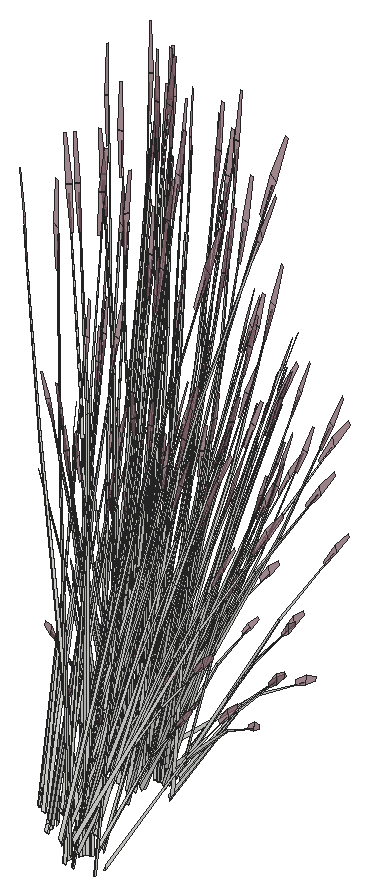
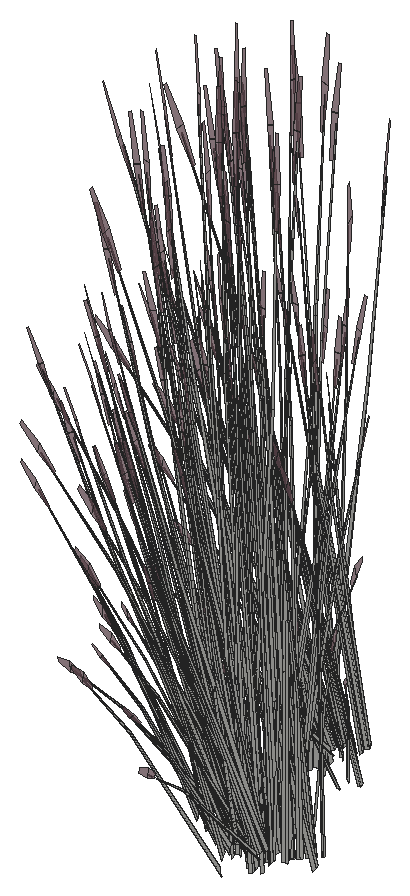
# SketchUp Ruby script. Lengths in inches.
U = 1.inch
M = Sketchup.active_model
def pt(a) = Geom::Point3d.new(a.map { |v| v * U })
def face(e, loops, mat)
  f = e.add_face(loops[0].map { |a| pt(a) })
  loops[1..].each { |l| e.add_face(l.map { |a| pt(a) }).erase! }
  f.material = f.back_material = mat if mat
  f
end
# faces: each face lists its corners as indices into pts; further lists are holes
def faces(e, pts, list, mat = nil) = list.each { |f| face(e, (f[0].is_a?(Array) ? f : [f]).map { |l| l.map { |i| pts[i] } }, mat) }
# xy, xz, yz: faces in a plane at the given z, y or x. An outline is a flat list of corners, or four numbers for a rectangle; further outlines are holes
def ring(l) = l.size == 4 ? [[l[0], l[1]], [l[2], l[1]], [l[2], l[3]], [l[0], l[3]]] : l.each_slice(2).to_a
def flat(e, list, mat, &to3) = list.each { |f| face(e, (f[0].is_a?(Array) ? f : [f]).map { |l| ring(l).map { |u, v| to3.(u, v) } }, mat) }
def xy(e, z, list, mat = nil) = flat(e, list, mat) { |x, y| [x, y, z] }
def xz(e, y, list, mat = nil) = flat(e, list, mat) { |x, z| [x, y, z] }
def yz(e, x, list, mat = nil) = flat(e, list, mat) { |y, z| [x, y, z] }
def lines(e, pts, list) = list.each { |a, b| e.add_line(pt(pts[a]), pt(pts[b])) }
# prism: a flat outline (further loops are holes) pulled along v
def prism(e, loops, v, mat = nil)
  f = face(e, loops, mat); d = Geom::Vector3d.new(v.map { |x| x * U })
  f.pushpull(f.normal.samedirection?(d) ? d.length : -d.length)
end
def box(e, o, s, mat = nil) = prism(e, [[o, [o[0] + s[0], o[1], o[2]], [o[0] + s[0], o[1] + s[1], o[2]], [o[0], o[1] + s[1], o[2]]]], [0, 0, s[2]], mat)
def at(x, y, z, deg = 0) = Geom::Transformation.translation(pt([x, y, z])) * Geom::Transformation.rotation(ORIGIN, Z_AXIS, deg.degrees)
def axes(o, x, y, z) = Geom::Transformation.new([*x, 0, *y, 0, *z, 0, *pt(o).to_a, 1])
def part(name) = M.definitions.add(name)
# library, detail: a bought-in or finely detailed component or shape, given as its bounding box
def library(name, o, s) = part(name).tap { |d| box(d.entities, o, s) }
def detail(e, o, s) = box(e.add_group.entities, o, s)
def put(e, d, t, mat = nil) = e.add_instance(d, t).tap { |i| i.material = mat if mat }
def group(e, t, mat = nil) = e.add_group.tap { |g| g.transformation = t; g.material = mat if mat }.entities
root = M.entities
M.materials.add("LightPink_Translucent").color = [144, 107, 117]
M.materials["LightPink_Translucent"].alpha = 0.75
c1 = part("blade")
p = [[2.15,0.21,22],[0,0.17,0],[0.09,0.45,0],[2.18,0.31,22],[2.29,0.31,22],[0.38,0.45,0],
  [2.48,0.24,33],[2.49,0.24,33],[2.48,0.22,33]]
faces(c1.entities,p,[[0,1,2,3],[4,5,2,3],[6,3,4,7],[8,0,3,6]])
c2 = part("seeds")
p = [[0.3,-0.1,1.38],[-0.01,-0.03,1.59],[-0.01,-0.03,0.03],[0.14,-0.07,-0.07],[0.29,-0.03,3],[0.15,0.01,3.11]]
faces(c2.entities,p,[[0,1,2,3],[1,0,4,5]],"LightPink_Translucent")
c3 = part("blade with seeds")
put(c3.entities,c1,at(0,0,0))
put(c3.entities,c2,axes([2.4,0.25,30.99],[1.5799,-0.05474,1.17369],[-0.12525,1.92788,0.29478],[-0.07173,-0.02425,1.56792]))
put(root,c3,axes([299.23,498.21,2.21],[-0.43405,0.58792,-0.44739],[-0.90188,-0.28295,0.21531],[0,0.13553,1.43643]))
put(root,c3,axes([301.09,499.59,4.73],[-0.65964,0.42992,0.48003],[-0.5689,-0.45657,0.3958],[0.30948,0.0793,0.9933]))
put(root,c3,axes([298.99,500.09,5.05],[-0.13817,-0.52554,0.35414],[0.78985,-0.13877,-0.4572],[0.21215,0.1506,0.87481]))
put(root,c3,axes([299.26,499.89,2.33],[1.11998,0.21207,0.30756],[-0.2802,0.75803,-0.36492],[-0.18537,0.09487,1.64885]))
put(root,c3,axes([299.18,500.41,2.02],[-0.83726,0.32623,-0.49651],[-0.50045,-0.58498,0],[-0.19069,0.0743,1.57504]))
put(root,c3,axes([301.96,498.47,2.02],[0,0.65246,-0.49651],[-1.00089,0,0],[0,0.1486,1.57504]))
put(root,c3,axes([299.46,498.55,3.875],[-0.3323,-0.11241,1.71376],[0.68769,-0.4716,0.13857],[0.42861,0.21275,0.73262]))
put(root,c3,axes([299.52,497.07,4.47],[-0.77304,-0.33901,1.38283],[0.81626,-0.52782,0.59665],[0.24941,0.31809,1.33663]))
put(root,c3,axes([300.6875,499.83,2.77],[-0.5037,-0.18761,1.1486],[0.6504,-0.19062,0.84392],[0.17543,0.16147,0.25299]))
put(root,c3,axes([298.92,500.36,5.03],[0.53309,-0.55848,-0.1216],[0.77201,0.32175,-0.67495],[0.26836,0.15779,1.02557]))
put(root,c3,axes([295.4,499.61,5.05],[0.60531,-0.34352,0.35414],[0.573,0.39225,-0.4572],[-0.08718,0.19929,0.87481]))
put(root,c3,axes([299.9375,500.3,2.375],[0.55932,0.6538,0],[-0.93577,0.36461,-0.51607],[-0.21313,0.08304,1.63711]))
put(root,c3,axes([298.22,500.83,4.71],[0.00265,-0.07899,1.77383],[0.76665,-0.34851,-0.16761],[0.2663,0.12439,0.31391]))
put(root,c3,axes([300.83,500.52,1.49],[0.06518,-0.0942,1.76342],[0.82057,-0.27742,-0.26939],[0.24877,0.14358,0.30037]))
put(root,c3,axes([299.46,497.72,2.84],[-0.02444,-0.61432,1.41272],[1.10603,0.15924,0.59816],[-0.26159,0.33615,1.3335]))
put(root,c3,axes([299.74,498.38,2.09],[0.32803,0.59738,-0.69212],[-0.94492,0.21515,-0.18165],[0.03626,0.20229,1.52773]))
put(root,c3,axes([299.55,500.09,4.68],[0.88277,-0.1551,-0.51099],[0.15442,0.58737,-0.3958],[0.23711,0.16832,0.97773]))
put(root,c3,axes([297.1,500.17,5.05],[0.2697,-0.50175,0.35414],[0.78684,0.14635,-0.4572],[0.07215,0.20201,0.87481]))
put(root,c3,axes([300.77,500.68,2.67],[-0.57368,-0.02046,1.0506],[0.37886,-0.43461,0.58006],[0.22663,0.15441,0.8241]))
put(root,c3,axes([299.11,500.57,4.73],[-0.4066,0.41448,0.0643],[-0.57901,-0.24131,0.50621],[0.18719,0.13288,0.77189]))
put(root,c3,axes([298.16,501.96,5.65],[0.61821,-0.37431,-0.06488],[0.56645,0.40995,-0.29416],[0.03988,0.11616,0.97024]))
put(root,c3,axes([299.28,500.45,4.73],[-0.88979,0.14973,0.48003],[-0.15442,-0.58737,0.3958],[0.20926,0.17311,0.9933]))
put(root,c3,axes([298.89,499.63,2.59],[0.01579,-0.21629,1.43002],[0.75442,-0.24159,-0.30754],[0.23289,0.25887,0.61141]))
put(root,c3,axes([296.85,500.63,4.73],[-0.6592,0.22175,0.0643],[-0.32265,-0.40436,0.50621],[0.06366,0.17825,0.77189]))
put(root,c3,axes([295.02,499.7,5.4],[0.98321,0.03233,-0.13498],[-0.02687,0.61208,-0.74919],[-0.0683,0.23574,1.13838]))
put(root,c3,axes([296.84,500.39,5.03],[0.87543,-0.30377,-0.1216],[0.4302,0.53915,-0.67495],[0.1155,0.2272,1.02557]))
put(root,c3,axes([294.42,509.26,2.59],[-0.25429,0.13207,1.43002],[-0.76157,-0.23115,-0.30754],[0.14117,-0.28747,0.61141]))
put(root,c3,axes([297.09,500.59,5.0625],[-0.88151,-0.17057,0.53283],[0.30143,-0.56078,0.43934],[0.05297,0.22053,1.10256]))
put(root,c3,axes([295.47,501.43,2.77],[-0.02315,-0.38796,1.1486],[0.57853,0.27671,0.84392],[-0.11378,0.18492,0.25299]))
put(root,c3,axes([296.99,500.5,1.49],[0.14478,-0.0355,1.76342],[0.8709,0.19542,-0.26939],[0.02547,0.22025,0.30037]))
put(root,c3,axes([295.6875,499.93,5],[0.64041,0.4384,-0.5672],[-0.67652,0.38394,-0.43934],[-0.09744,0.22274,1.08528]))
put(root,c3,axes([295.04,510.24,4.98],[0.02328,-0.60353,-0.71045],[0.98022,0.04053,0.08574],[0.10344,-0.25568,1.00501]))
put(root,c3,axes([294.99,500.59,2.82],[0.8127,-0.11554,0.06507],[0.18684,0.46549,-0.86304],[-0.05152,0.23564,0.7736]))
put(root,c3,axes([297.59,500.36,4.68],[0.87941,0.16356,-0.51099],[-0.30143,0.56078,-0.3958],[0.08064,0.22578,0.97773]))
put(root,c3,axes([298.09,499.2,3.875],[-0.2045,-0.20949,1.71376],[0.94495,-0.17636,0.13857],[0.21357,0.32887,0.73262]))
put(root,c3,axes([296.4,509.3,4.72],[-0.00864,-0.12985,1.74944],[-0.72937,-0.3753,-0.27667],[0.11277,-0.2275,0.14031]))
put(root,c3,axes([293.93,509.93,3.875],[-0.16657,0.22426,1.71376],[-0.69879,-0.4641,0.13857],[0.31524,-0.28926,0.73262]))
put(root,c3,axes([296.21,508.83,4.71],[-0.09085,0.04984,1.77383],[-0.89014,-0.16814,-0.16761],[-0.03222,-0.21748,0.31391]))
put(root,c3,axes([297.1875,500.7,4.53],[-0.2697,0.50175,-0.35414],[-0.78684,-0.14635,0.4572],[0.07215,0.20201,0.87481]))
put(root,c3,axes([293.48,508.21,2.77],[0.11476,0.38047,1.1486],[-0.63664,-0.21072,0.84392],[0.06851,-0.19481,0.25299]))
put(root,c3,axes([295.49,499.73,5.34],[-0.02328,0.60353,-0.7886],[-0.98022,-0.04053,0.09517],[-0.10344,0.25568,1.11556]))
put(root,c3,axes([294.84,510.04,4.68],[-0.64041,-0.4384,-0.51099],[0.67652,-0.38394,-0.3958],[0.09744,-0.22274,0.97773]))
put(root,c3,axes([296.42,499.3,3.875],[-0.0219,-0.25042,1.71376],[0.94901,0.16613,0.13857],[-0.0587,0.35688,0.73262]))
put(root,c3,axes([297.27,500.25,4.98],[0.42698,0.53052,-0.71045],[-0.87893,0.29566,0.08574],[0.09984,0.25633,1.00501]))
put(root,c3,axes([293.4375,509.39,4.73],[0.88151,0.17057,0.48003],[-0.30143,0.56078,0.3958],[-0.05297,-0.22053,0.9933]))
put(root,c3,axes([295.51,510.27,5.03],[-0.98321,-0.03233,-0.1216],[0.02687,-0.61208,-0.67495],[0.0683,-0.23574,1.02557]))
put(root,c3,axes([295.44,509.875,4.53],[0.60531,-0.34352,-0.35414],[0.573,0.39225,0.4572],[0.08718,-0.19929,0.87481]))
put(root,c3,axes([293.67,509.34,4.73],[0.6592,-0.22175,0.0643],[0.32265,0.40436,0.50621],[-0.06366,-0.17825,0.77189]))
put(root,c3,axes([296.63,501.59,4.72],[0.1134,0.10507,1.74944],[0.91515,0.04128,-0.27667],[0.09203,0.23172,0.14031]))
put(root,c3,axes([295.16,500.58,3.36],[0.01966,-0.33682,1.54345],[0.88405,0.17791,0.21329],[-0.0766,0.35897,0.72882]))
put(root,c3,axes([296.2,509.67,1.49],[-0.1339,-0.0514,1.76342],[-0.34394,-0.57425,-0.26939],[0.23202,-0.15583,0.30037]))
put(root,c3,axes([295.4375,510.01,4.73],[0.63704,0.44518,0.48003],[-0.67652,0.38394,0.3958],[0.11751,-0.20886,0.9933]))
put(root,c3,axes([295.67,510.05,4.73],[0.73517,0.0304,0.0643],[-0.02016,0.45906,0.50621],[0.07693,-0.17585,0.77189]))
put(root,c3,axes([295.125,510.36,5.05],[-0.60531,0.34352,0.35414],[-0.573,-0.39225,-0.4572],[0.08718,-0.19929,0.87481]))
put(root,c3,axes([296.19,511.29,4.98],[0.4673,-0.51481,-0.71045],[0.81887,0.36587,0.08574],[0.27902,-0.18652,1.00501]))
put(root,c3,axes([291.14,509.79,2.375],[-0.55932,-0.6538,0],[0.93577,-0.36461,-0.51607],[0.21313,-0.08304,1.63711]))
put(root,c3,axes([296.17,511.05,4.68],[-0.22982,-0.59576,-0.51099],[0.87033,-0.10422,-0.3958],[0.24941,-0.16002,0.97773]))
put(root,c3,axes([296.58,511.47,5.03],[-0.82753,-0.35977,-0.1216],[0.47675,-0.52101,-0.67495],[0.2338,-0.18111,1.02557]))
put(root,c3,axes([291.9,509.6875,2.02],[0.83726,-0.32623,-0.49651],[0.50045,0.58498,0],[0.19069,-0.0743,1.57504]))
put(root,c3,axes([296.87,510.82,2.59],[-0.31959,-0.01933,1.43002],[-0.32741,-0.51843,-0.30754],[0.39262,-0.14666,0.61141]))
put(root,c3,axes([298.62,511.32,4.71],[-0.11685,-0.00496,1.77383],[-0.48522,-0.53096,-0.16761],[0.19486,-0.17458,0.31391]))
put(root,c3,axes([292.89,511.03,2.06],[0.60257,-0.49041,-0.62353],[0.74854,0.44469,-0.16365],[0.24146,-0.12234,1.37633]))
put(root,c3,axes([297.24,509.86,2.77],[-0.29798,0.33213,1.1486],[-0.25612,-0.44624,0.84392],[0.24611,-0.11182,0.25299]))
put(root,c3,axes([296.8125,511.11,4.53],[0.77872,-0.09325,-0.35414],[0.20563,0.53305,0.4572],[0.22316,-0.14318,0.87481]))
put(root,c3,axes([292.24,511.59,2.67],[-0.10425,-0.7445,-0.29095],[1.08575,-0.04502,-0.50002],[0.19119,-0.09917,1.59708]))
put(root,c3,axes([296.18,511.43,5.05],[-0.77872,0.09325,0.35414],[-0.20563,-0.53305,-0.4572],[0.22316,-0.14318,0.87481]))
put(root,c3,axes([292.1,509.95,2.03],[0.83462,0.16144,-0.30978],[-0.21015,0.56852,0.30978],[0.16826,-0.06556,1.38974]))
put(root,c3,axes([296.88,511.34,4.73],[0.61415,0.2744,0.0643],[-0.35756,0.39076,0.50621],[0.1969,-0.12633,0.77189]))
put(root,c3,axes([296.71,511.23,4.73],[0.22187,0.60049,0.48003],[-0.87033,0.10422,0.3958],[0.25651,-0.14123,0.9933]))
put(root,c3,axes([299.06,511.95,4.72],[0.12414,-0.09938,1.74944],[-0.15889,-0.60963,-0.27667],[0.31148,-0.11559,0.14031]))
put(root,c3,axes([292.38,512.18,2.43],[1.00799,0.31623,0.24065],[-0.48511,0.65709,0.50002],[0,-0.15147,1.60543]))
put(root,c3,axes([292.06,511.74,2.72],[-0.97146,0.04028,0.44739],[-0.08785,-0.66859,-0.21531],[0.17391,-0.06776,1.43643]))
put(root,c3,axes([296.61,512.88,5.03],[-0.45012,-0.59081,-0.1216],[0.79888,-0.29033,-0.67495],[0.33665,-0.07795,1.02557]))
put(root,c3,axes([296.57,512.37,4.68],[0.24236,-0.59349,-0.51099],[0.83094,0.20343,-0.3958],[0.33455,-0.05442,0.97773]))
put(root,c3,axes([295.26,509.95,2.375],[0.55932,-0.6538,0],[0.93577,0.36461,-0.51607],[0.21313,0.08304,1.63711]))
put(root,c3,axes([297.46,512.54,1.98],[-0.57619,0.0783,1.41583],[-0.09171,-0.62326,0.08104],[0.40356,-0.09434,0.80566]))
put(root,c3,axes([298.51,511.99,2.26],[-0.55463,-0.41721,-0.06488],[0.60744,-0.38228,-0.29416],[0.17212,-0.02691,0.97024]))
put(root,c3,axes([293.42,512.04,2.21],[0,-0.75495,0],[1.11865,0,0],[0,0,1.79456]))
put(root,c3,axes([294.78,510.3,2.48],[-0.83726,-0.32623,0.49651],[0.50045,-0.58498,0],[0.19069,0.0743,1.57504]))
put(root,c3,axes([296.41,512.59,4.98],[0.78611,-0.28816,-0.71045],[0.4381,0.59317,0.08574],[0.37982,-0.06738,1.00501]))
put(root,c3,axes([292.89,511.56,2.36],[-0.74176,0.59212,0.45755],[-0.88124,-0.52269,0.17955],[0.17882,-0.05909,1.58856]))
put(root,c3,axes([291.6,510.59,2.47],[-0.25843,0.64844,0.17642],[-0.9457,-0.1835,0.35086],[0.16336,-0.00316,1.60407]))
put(root,c3,axes([296.3,512.7,5.05],[-0.74348,-0.18202,0.35414],[0.21685,-0.53102,-0.4572],[0.29933,-0.04869,0.87481]))
put(root,c3,axes([291.21,511.11,1.59],[-0.88056,0.26122,1.28929],[-0.28027,-0.74951,0.50096],[0.54072,0.01247,1.46642]))
put(root,c3,axes([293.58,511.3125,2.62],[0.17258,-0.58229,0.1448],[0.84319,0.10108,-0.41347],[0.15345,0.05979,1.26744]))
put(root,c3,axes([298.09,512.13,1.49],[-0.04675,-0.09906,1.76342],[0.32428,-0.57943,-0.26939],[0.32711,-0.00833,0.30037]))
put(root,c3,axes([293.22,511.46,2.72],[-0.53742,-0.54764,0.44739],[0.81403,-0.38564,-0.21531],[0.17391,0.06776,1.43643]))
put(root,c3,axes([293.49,511.5,2.67],[0.90324,-0.43318,-0.29095],[0.60064,0.61207,-0.50002],[0.22285,0.06216,1.59708]))
put(root,c3,axes([297.08,512.64,4.53],[0.74348,0.18202,-0.35414],[-0.21685,0.53102,0.4572],[0.29933,-0.04869,0.87481]))
put(root,c3,axes([295.77,510.35,2.02],[0.83726,0.32623,-0.49651],[-0.50045,0.58498,0],[0.19069,0.0743,1.57504]))
put(root,c3,axes([294.18,512.21,2.21],[1.00089,0,0],[0,0.67548,0],[0,0,1.78407]))
put(root,c3,axes([294.46,510.625,2.47],[-0.96132,0.17317,0.17642],[-0.23737,-0.64447,0.35086],[0.08574,0.0939,1.60407]))
put(root,c3,axes([295.06,511.98,3.875],[-0.37107,0.01478,1.71376],[0.24616,-0.64047,0.13857],[0.5288,0.03961,0.73262]))
put(root,c3,axes([295.54,510.59,2.03],[0.21015,0.56852,-0.30978],[-0.83462,0.16144,0.30978],[0.16826,0.06556,1.38974]))
put(root,c3,axes([296.97,512.87,4.73],[0.32857,0.44488,0.0643],[-0.59916,0.21775,0.50621],[0.26412,-0.04296,0.77189]))
put(root,c3,axes([293.86,511.87,2.38],[-1.13071,-0.13747,0.49198],[0.23011,-0.77639,0.19306],[0.16524,0.07497,1.70813]))
put(root,c3,axes([296.91,512.71,4.73],[-0.25275,0.59491,0.48003],[-0.83094,-0.20343,0.3958],[0.32677,-0.03575,0.9933]))
put(root,c3,axes([294.05,513.7,2.18],[0.93921,-0.22138,-0.19198],[0.33003,0.6377,0.00008],[0.10367,-0.02447,1.73897]))
put(root,c3,axes([294.16,512.5,2.21],[0.62448,0.42144,0],[-0.62448,0.42144,0],[0,0,1.69266]))
put(root,c3,axes([295.85,512.32,2.47],[-0.70288,-0.47526,0.17642],[0.70832,-0.46097,0.35086],[-0.07763,0.09706,1.60407]))
put(root,c3,axes([294.55,511.6,2.06],[0.9306,0.10697,-0.62353],[-0.19638,0.65984,-0.16365],[0.27771,0.07995,1.37633]))
put(root,c3,axes([298.66,512.75,2.77],[-0.55274,0.10771,1.1486],[0.26018,-0.44517,0.84392],[0.29323,0.03046,0.25299]))
put(root,c3,axes([294.15,512.01,2.72],[0.43405,-0.58792,0.44739],[0.90188,0.28295,-0.21531],[0,0.13553,1.43643]))
put(root,c3,axes([298.4,514.63,4.71],[-0.08089,-0.05712,1.77383],[0.17695,-0.61228,-0.16761],[0.31864,-0.03912,0.31391]))
put(root,c3,axes([293.98,512.34,2.29],[0,0.75458,-0.05637],[-1.11865,0,0],[0,0.02371,1.79368]))
put(root,c3,axes([294.06,511.81,2.21],[0.53742,0.54764,-0.44739],[-0.81403,0.38564,0.21531],[0.17391,0.06776,1.43643]))
put(root,c3,axes([297.7,514.12,3.93],[-0.17122,-0.54847,-0.03492],[0.80929,-0.12609,-0.15832],[0.169,0.03477,0.52218]))
put(root,c3,axes([295.6,514.11,5.03],[0.0479,-0.66354,-0.1216],[0.90696,0.01814,-0.67495],[0.3493,0.04609,1.02557]))
put(root,c3,axes([296.43,512.33,2.48],[0,-0.65246,0.49651],[1.00089,0,0],[0,0.1486,1.57504]))
put(root,c3,axes([294.53,512.14,2.62],[0.83351,-0.19028,0.1448],[0.29189,0.54335,-0.41347],[0,0.11958,1.26744]))
put(root,c3,axes([295.46,513.85,5.05],[-0.50902,-0.40851,0.35414],[0.58122,-0.38671,-0.4572],[0.29531,0.05884,0.87481]))
put(root,c3,axes([297.625,513.46,2.59],[-0.21545,-0.16047,1.43002],[0.28033,-0.53085,-0.30754],[0.43591,0.07191,0.61141]))
put(root,c3,axes([293.77,514.05,2.2],[0.90188,0.29293,0],[-0.43405,0.60866,0],[0,0,1.74954]))
put(root,c3,axes([296.39,513.71,4.72],[0.19191,-0.01103,1.74944],[0.52639,-0.5069,-0.27667],[0.34136,0.06691,0.14031]))
put(root,c3,axes([295.65,513.79,4.98],[0.89428,0.01571,-0.71045],[-0.06006,0.66153,0.08574],[0.37886,0.06981,1.00501]))
put(root,c3,axes([293.45,513.8,2.29],[0.38895,0.74956,-0.06012],[-1.11135,0.26265,0],[0.01358,0.02618,1.72173]))
put(root,c3,axes([297.11,512.44,2.375],[1.11865,0,0],[0,0.72922,-0.51607],[0,0.16609,1.63711]))
put(root,c3,axes([296.66,512.82,2.2],[-1.1181,-0.00522,-0.04976],[0,-0.72922,0.49943],[-0.03514,0.166,1.58352]))
put(root,c3,axes([294.24,512.18,2.67],[1.00749,0.31132,-0.29095],[-0.48511,0.65709,-0.50002],[0.03166,0.16133,1.59708]))
put(root,c3,axes([296.18,514.06,4.53],[0.50902,0.40851,-0.35414],[-0.58122,0.38671,0.4572],[0.29531,0.05884,0.87481]))
put(root,c3,axes([296.43,512.92,2.03],[-0.62448,0.40708,-0.30978],[-0.62448,-0.40708,0.30978],[0,0.13112,1.38974]))
put(root,c3,axes([295.92,514.22,4.73],[-0.04505,0.49615,0.0643],[-0.68022,-0.0136,0.50621],[0.26056,0.05192,0.77189]))
put(root,c3,axes([294.13,512.67,2.21],[-0.43405,0.58792,-0.44739],[-0.90188,-0.28295,0.21531],[0,0.13553,1.43643]))
put(root,c3,axes([295.99,514.06,4.73],[-0.65964,0.42992,0.48003],[-0.5689,-0.45657,0.3958],[0.30948,0.0793,0.9933]))
put(root,c3,axes([293.89,514.56,5.05],[-0.13817,-0.52554,0.35414],[0.78985,-0.13877,-0.4572],[0.21215,0.1506,0.87481]))
put(root,c3,axes([296.86,512.9375,2.02],[0,0.65246,-0.49651],[-1.00089,0,0],[0,0.1486,1.57504]))
put(root,c3,axes([294.36,513.01,3.875],[-0.3323,-0.11241,1.71376],[0.68769,-0.4716,0.13857],[0.42861,0.21275,0.73262]))
put(root,c3,axes([294.42,511.53,4.47],[-0.77304,-0.33901,1.38283],[0.81626,-0.52782,0.59665],[0.24941,0.31809,1.33663]))
put(root,c3,axes([295.59,514.29,2.77],[-0.5037,-0.18761,1.1486],[0.6504,-0.19062,0.84392],[0.17543,0.16147,0.25299]))
put(root,c3,axes([293.82,514.83,5.03],[0.53309,-0.55848,-0.1216],[0.77201,0.32175,-0.67495],[0.26836,0.15779,1.02557]))
put(root,c3,axes([293.12,515.29,4.71],[0.00265,-0.07899,1.77383],[0.76665,-0.34851,-0.16761],[0.2663,0.12439,0.31391]))
put(root,c3,axes([295.73,514.99,1.49],[0.06518,-0.0942,1.76342],[0.82057,-0.27742,-0.26939],[0.24877,0.14358,0.30037]))
put(root,c3,axes([294.64,512.85,2.09],[0.32803,0.59738,-0.69212],[-0.94492,0.21515,-0.18165],[0.03626,0.20229,1.52773]))
put(root,c3,axes([294.45,514.55,4.68],[0.88277,-0.1551,-0.51099],[0.15442,0.58737,-0.3958],[0.23711,0.16832,0.97773]))
put(root,c3,axes([292,514.64,5.05],[0.2697,-0.50175,0.35414],[0.78684,0.14635,-0.4572],[0.07215,0.20201,0.87481]))
put(root,c3,axes([295.67,515.15,2.67],[-0.57368,-0.02046,1.0506],[0.37886,-0.43461,0.58006],[0.22663,0.15441,0.8241]))
put(root,c3,axes([294.01,515.03,4.73],[-0.4066,0.41448,0.0643],[-0.57901,-0.24131,0.50621],[0.18719,0.13288,0.77189]))
put(root,c3,axes([293.06,516.43,5.65],[0.61821,-0.37431,-0.06488],[0.56645,0.40995,-0.29416],[0.03988,0.11616,0.97024]))
put(root,c3,axes([294.18,514.92,4.73],[-0.88979,0.14973,0.48003],[-0.15442,-0.58737,0.3958],[0.20926,0.17311,0.9933]))
put(root,c3,axes([293.79,514.09,2.59],[0.01579,-0.21629,1.43002],[0.75442,-0.24159,-0.30754],[0.23289,0.25887,0.61141]))
put(root,c3,axes([291.74,514.85,5.03],[0.87543,-0.30377,-0.1216],[0.4302,0.53915,-0.67495],[0.1155,0.2272,1.02557]))
put(root,c3,axes([292.49,514.82,4.68],[0.87941,0.16356,-0.51099],[-0.30143,0.56078,-0.3958],[0.08064,0.22578,0.97773]))
put(root,c3,axes([292.99,513.67,3.875],[-0.2045,-0.20949,1.71376],[0.94495,-0.17636,0.13857],[0.21357,0.32887,0.73262]))
put(root,c3,axes([292.17,514.72,4.98],[0.42698,0.53052,-0.71045],[-0.87893,0.29566,0.08574],[0.09984,0.25633,1.00501]))
put(root,c3,axes([291.53,516.06,4.72],[0.1134,0.10507,1.74944],[0.91515,0.04128,-0.27667],[0.09203,0.23172,0.14031]))
